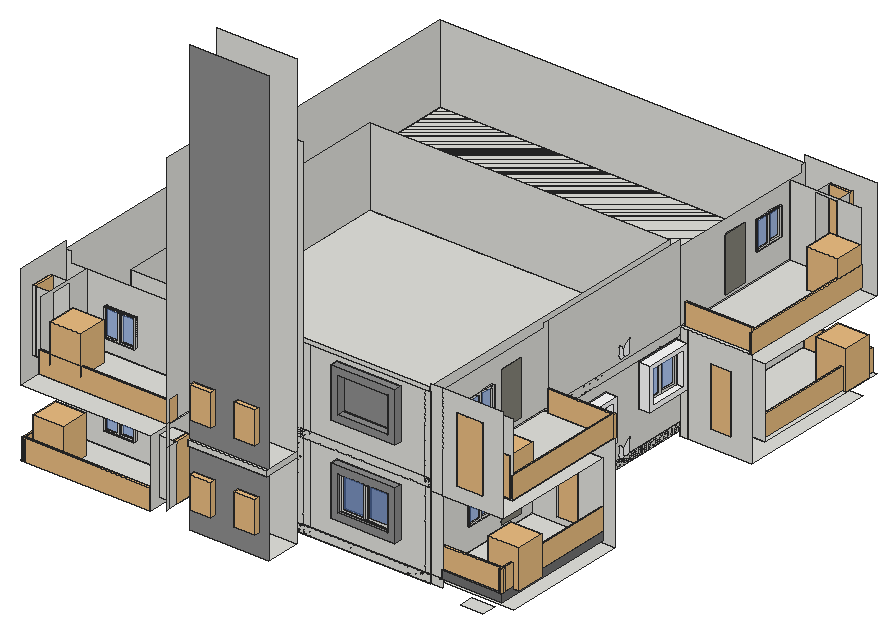
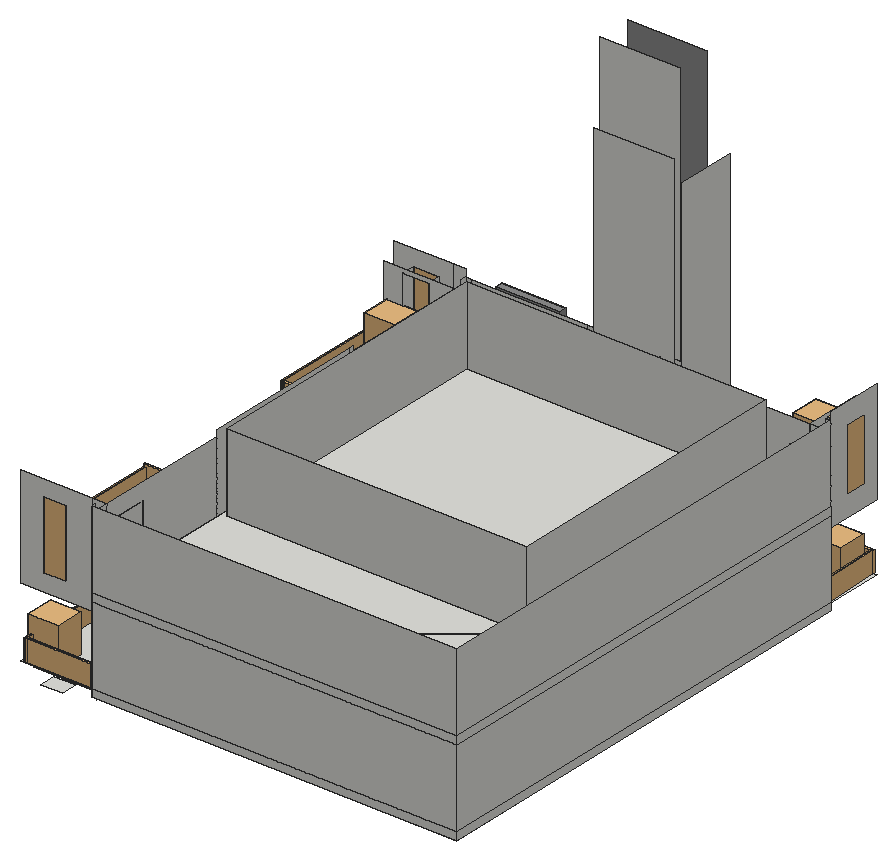
# SketchUp Ruby script. Lengths in inches.
U = 1.inch
M = Sketchup.active_model
def pt(a) = Geom::Point3d.new(a.map { |v| v * U })
def face(e, loops, mat)
  f = e.add_face(loops[0].map { |a| pt(a) })
  loops[1..].each { |l| e.add_face(l.map { |a| pt(a) }).erase! }
  f.material = f.back_material = mat if mat
  f
end
# faces: each face lists its corners as indices into pts; further lists are holes
def faces(e, pts, list, mat = nil) = list.each { |f| face(e, (f[0].is_a?(Array) ? f : [f]).map { |l| l.map { |i| pts[i] } }, mat) }
# xy, xz, yz: faces in a plane at the given z, y or x. An outline is a flat list of corners, or four numbers for a rectangle; further outlines are holes
def ring(l) = l.size == 4 ? [[l[0], l[1]], [l[2], l[1]], [l[2], l[3]], [l[0], l[3]]] : l.each_slice(2).to_a
def flat(e, list, mat, &to3) = list.each { |f| face(e, (f[0].is_a?(Array) ? f : [f]).map { |l| ring(l).map { |u, v| to3.(u, v) } }, mat) }
def xy(e, z, list, mat = nil) = flat(e, list, mat) { |x, y| [x, y, z] }
def xz(e, y, list, mat = nil) = flat(e, list, mat) { |x, z| [x, y, z] }
def yz(e, x, list, mat = nil) = flat(e, list, mat) { |y, z| [x, y, z] }
def lines(e, pts, list) = list.each { |a, b| e.add_line(pt(pts[a]), pt(pts[b])) }
# prism: a flat outline (further loops are holes) pulled along v
def prism(e, loops, v, mat = nil)
  f = face(e, loops, mat); d = Geom::Vector3d.new(v.map { |x| x * U })
  f.pushpull(f.normal.samedirection?(d) ? d.length : -d.length)
end
def box(e, o, s, mat = nil) = prism(e, [[o, [o[0] + s[0], o[1], o[2]], [o[0] + s[0], o[1] + s[1], o[2]], [o[0], o[1] + s[1], o[2]]]], [0, 0, s[2]], mat)
def at(x, y, z, deg = 0) = Geom::Transformation.translation(pt([x, y, z])) * Geom::Transformation.rotation(ORIGIN, Z_AXIS, deg.degrees)
def axes(o, x, y, z) = Geom::Transformation.new([*x, 0, *y, 0, *z, 0, *pt(o).to_a, 1])
def part(name) = M.definitions.add(name)
# library, detail: a bought-in or finely detailed component or shape, given as its bounding box
def library(name, o, s) = part(name).tap { |d| box(d.entities, o, s) }
def detail(e, o, s) = box(e.add_group.entities, o, s)
def put(e, d, t, mat = nil) = e.add_instance(d, t).tap { |i| i.material = mat if mat }
def group(e, t, mat = nil) = e.add_group.tap { |g| g.transformation = t; g.material = mat if mat }.entities
root = M.entities
M.materials.add("[Color C05]").color = [255, 127, 0]
M.materials.add("[Color M00]").color = [255, 255, 255]
M.materials.add("[Color M04]").color = [142, 142, 142]
M.materials.add("[Color M05]").color = [114, 114, 114]
M.materials.add("[Translucent Glass Blue]").color = [100, 149, 237]
M.materials["[Translucent Glass Blue]"].alpha = 0.5
M.materials.add("pic").color = [134, 132, 121]
c1 = library("KentiaPalm",[-22.86,-14.31,0],[47.49,43.96,59.125])
c2 = library("grade+varanda",[25.2,-1.57,0],[92.91,3.14,40.94])
c3 = part("Door leaf")
xy(c3.entities,0,[[0,0,28.74,2]],"pic")
xy(c3.entities,75.2,[[0,0,28.74,2]],"pic")
xz(c3.entities,0,[[0,0,28.74,75.2]],"pic")
xz(c3.entities,2,[[0,0,28.74,75.2]],"pic")
yz(c3.entities,0,[[0,0,2,75.2]])
yz(c3.entities,28.74,[[0,0,2,75.2]])
c4 = library("CNC CUTTING TEXTURE",[0,0,-0.79],[85.98,295.47,0.79])
c5 = library("Framed window",[0,0,0],[23.62,8.27,35.43])
c6 = part("Janela aluminio")
xy(c6.entities,0,[[0,0,47.24,1.57],[23.62,1.57,47.24,2.76],[0,2.76,25.98,3.9375],[0,3.9375,47.24,5.91]])
xy(c6.entities,43.31,[[0,0,47.24,1.57],[23.62,1.57,47.24,2.76],[0,2.76,0,5.91,47.24,5.91,47.24,3.9375,25.98,3.9375,25.98,2.76],[25.98,2.76,47.24,3.9375]])
xz(c6.entities,1.57,[[0,0,23.62,0,23.62,41.34,21.26,41.34,21.26,1.97,1.97,1.97,1.97,41.34,23.62,41.34,23.62,43.31,0,43.31],[[23.62,0,47.24,43.31],[25.7,1.97,45.28,41.34]]])
xz(c6.entities,2.76,[[[0,0,23.62,43.31],[2.36,2.36,21.26,40.94]],[23.62,0,25.98,43.31]])
xz(c6.entities,2.76,[[2.36,2.36,21.26,40.94]],"[Translucent Glass Blue]")
xz(c6.entities,3.9375,[[25.98,0,25.98,2.36,44.88,2.36,44.88,40.94,25.98,40.94,25.98,43.31,47.24,43.31,47.24,0]])
xz(c6.entities,3.9375,[[25.98,2.36,44.88,40.94]],"[Translucent Glass Blue]")
yz(c6.entities,0,[[0,0,1.57,43.31],[2.76,0,5.91,43.31]])
yz(c6.entities,23.62,[[1.57,0,2.76,43.31]])
yz(c6.entities,25.98,[[2.76,0,3.9375,43.31]])
yz(c6.entities,47.24,[[0,0,1.57,43.31],[1.57,0,2.76,43.31],[3.9375,0,5.91,43.31]])
c7 = part("Group\#81")
xy(c7.entities,0,[[[0,0,99.375,76.3125],[10.74,10.74,88.63,65.57]],[10.74,10.74,88.63,65.57]])
xy(c7.entities,11.8125,[[[0,0,99.375,76.3125],[10.74,10.74,88.63,65.57]]])
xz(c7.entities,0,[[0,0,99.375,11.8125]])
xz(c7.entities,10.74,[[10.74,0,88.63,11.8125]])
xz(c7.entities,65.57,[[10.74,0,88.63,11.8125]])
xz(c7.entities,76.3125,[[0,0,99.375,11.8125]])
yz(c7.entities,0,[[0,0,76.3125,11.8125]])
yz(c7.entities,10.74,[[10.74,0,65.57,11.8125]])
yz(c7.entities,88.63,[[10.74,0,65.57,11.8125]])
yz(c7.entities,99.375,[[0,0,76.3125,11.8125]])
c8 = part("Group\#73")
xy(c8.entities,0,[[6.22,6.22,66.16,57.66]],"[Color M00]")
xy(c8.entities,0,[[[0,0,72.375,63.875],[6.22,6.22,66.16,57.66]]],"[Color M04]")
xy(c8.entities,16.6875,[[[0,0,72.375,63.875],[6.22,6.22,66.16,57.66]]],"[Color M00]")
xz(c8.entities,0,[[0,0,72.375,16.6875]],"[Color M00]")
xz(c8.entities,6.22,[[6.22,0,66.16,16.6875]],"[Color M00]")
xz(c8.entities,57.66,[[6.22,0,66.16,16.6875]],"[Color M04]")
xz(c8.entities,63.875,[[0,0,72.375,16.6875]],"[Color M00]")
yz(c8.entities,0,[[0,0,63.875,16.6875]],"[Color M00]")
yz(c8.entities,6.22,[[6.22,0,57.66,16.6875]],"[Color M00]")
yz(c8.entities,66.16,[[6.22,0,57.66,16.6875]],"[Color M00]")
yz(c8.entities,72.375,[[0,0,63.875,16.6875]],"[Color M00]")
xy(root,277.65,[[815.15,221.79,849.53,244.2]])
xy(root,281.18,[[448.85,157.26,571.01,210.63]])
xy(root,281.29,[[813.66,917.62,847.23,942.88]])
xy(root,283.71,[[769.63,702.05,769.63,917.62,879.32,917.62,879.32,702.13,780.63,702.13,780.63,702.05]])
xy(root,284.02,[[769.63,244.2,879.32,439.19]])
xy(root,291.08,[[[206.95,222.13,769.63,942.88],[298.63,231.13,760.63,693.13]]])
xy(root,303.08,[[206.95,133.63,408.57,222.13],[769.63,221.79,786.7,222.13],[786.7,221.79,879.32,221.79,879.32,415.6,867.32,415.6,867.32,232.67,786.7,232.67],[[206.95,222.13,769.63,942.88],[298.63,231.13,760.63,693.13]],[769.63,222.13,786.7,222.13,786.7,232.67,867.32,232.67,867.32,415.6,769.63,415.6],
  [298.63,231.13,760.63,693.13],[769.63,728.91,879.32,942.88]])
xy(root,310.63,[[816.63,702.13,847.63,728.91]])
xy(root,311.64,[[808.92,415.6,840.79,439.19]])
xy(root,315.48,[[408.57,149.23,436.38,173.48]])
xy(root,316.02,[[786.7,221.79,879.32,221.79,879.32,415.6,867.32,415.6,867.32,232.67,786.7,232.67]],"[Color M05]")
xy(root,399.95,[[816.63,702.13,847.63,728.91]])
xy(root,402.1,[[408.57,149.23,436.38,173.48]])
xy(root,406.33,[[206.95,133.63,408.57,222.13]])
xy(root,407.95,[[808.92,415.6,840.79,439.19]])
xy(root,410.02,[[769.63,728.91,879.32,942.88]])
xy(root,418.39,[[769.63,222.13,879.32,415.6]])
xy(root,423.08,[[[206.95,222.13,769.63,942.88],[298.63,231.13,760.63,693.13]]])
xy(root,435.08,[[237.95,133.63,436.38,222.13],[[206.95,222.13,769.63,942.88],[298.63,231.13,760.63,693.13]],[298.63,231.13,760.63,693.13],[769.63,242.1,879.32,439.19],[769.63,702.05,780.63,702.05,780.63,702.13,879.32,702.13,879.32,913.11,769.63,913.11]])
xy(root,437.55,[[809.28,913.11,842.4,942.88]])
xy(root,438.3,[[206.95,156.57,237.95,190.94]])
xy(root,440.0625,[[810.64,222.13,849.77,242.1]])
xz(root,149.23,[[408.57,315.48,436.38,402.1]])
xz(root,156.57,[[206.95,438.3,237.95,534.42]])
xz(root,157.26,[[448.85,281.18,571.01,951.08]],"[Color M04]")
xz(root,173.48,[[408.57,315.48,436.38,402.1]])
xz(root,190.94,[[206.95,438.3,237.95,534.42]])
xz(root,210.63,[[448.85,281.18,571.01,951.08]])
xz(root,221.79,[[786.7,303.08,879.32,316.02]],"[Color M05]")
xz(root,222.13,[[206.95,291.08,436.38,303.08],[436.38,291.08,448.85,303.08],[448.85,291.08,571.01,831.08],[571.01,291.08,582.45,303.08],[582.45,291.08,759.63,303.08],
  [759.63,291.08,787.51,303.08],[206.95,303.08,408.57,406.33],[408.57,303.08,436.38,303.08,436.38,423.08,425.76,423.08,425.76,406.33,408.57,406.33],[436.38,303.08,448.85,423.08],[448.85,303.08,571.01,423.08],
  [571.01,303.08,582.45,423.08],[582.45,303.08,759.63,423.08],[759.63,303.08,769.63,423.08],[769.63,303.08,787.51,418.39],[206.95,406.33,425.76,423.08],
  [769.63,418.39,787.51,567.08],[[787.51,418.39,879.32,567.08],[810.64,440.0625,849.77,541.5625]],[206.95,423.08,436.38,435.08],[436.38,423.08,448.85,435.08],[571.01,423.08,582.45,435.08],
  [582.45,423.08,759.63,435.08],[759.63,423.08,769.63,435.08],[206.95,435.08,237.95,435.08,237.95,538.83,213.89,538.83,213.89,555.08,206.95,555.08],[237.95,435.08,436.38,435.08,436.38,555.08,435.45,555.08,435.45,538.83,237.95,538.83],[436.38,435.08,448.85,555.08],
  [448.85,435.08,571.01,555.08],[571.01,435.08,582.45,555.08],[582.45,435.08,759.63,555.08],[759.63,435.08,769.63,555.08]])
xz(root,231.13,[[298.63,303.08,760.63,423.08],[298.63,435.08,760.63,555.08]])
xz(root,232.67,[[786.7,303.08,867.32,316.02]])
xz(root,242.1,[[[769.63,435.08,879.32,548.14],[810.64,440.0625,849.77,541.5625]]])
xz(root,415.6,[[[769.63,303.08,867.32,303.08,867.32,316.02,879.32,316.02,879.32,418.39,769.63,418.39],[808.92,311.64,840.79,407.95]],[867.32,303.08,879.32,316.02]])
xz(root,439.19,[[[769.63,284.02,879.32,435.08],[808.92,311.64,840.79,407.95]]])
xz(root,693.13,[[298.63,303.08,760.63,423.08],[298.63,435.08,760.63,555.08]])
xz(root,702.05,[[769.63,283.71,780.63,435.08]])
xz(root,702.13,[[[780.63,283.71,879.32,435.08],[816.63,310.63,847.63,399.95]]])
xz(root,728.91,[[[769.63,303.08,879.32,410.02],[816.63,310.63,847.63,399.95]]])
xz(root,913.11,[[[769.63,435.08,879.32,545.21],[809.28,437.55,842.4,541.92]]])
xz(root,942.88,[[206.95,303.08,769.63,423.08],[[769.63,410.02,879.32,567.08],[809.28,437.55,842.4,541.92]],[206.95,435.08,769.63,555.08]])
yz(root,206.95,[[222.13,303.08,942.88,423.08],[[133.63,406.33,222.13,567.08],[156.57,438.3,190.94,534.42]],[222.13,435.08,942.88,555.08]])
yz(root,237.95,[[[133.63,435.08,222.13,538.83],[156.57,438.3,190.94,534.42]]])
yz(root,298.63,[[231.13,303.08,693.13,423.08],[231.13,435.08,693.13,555.08]])
yz(root,408.57,[[[133.63,303.08,222.13,406.33],[149.23,315.48,173.48,402.1]]])
yz(root,436.38,[[129.69,315.48,133.63,402.1],[133.63,315.48,149.23,402.1],[149.23,315.48,173.48,402.1],[129.69,402.1,133.63,435.08],[129.69,435.08,222.13,802.33]])
yz(root,760.63,[[231.13,303.08,693.13,423.08],[231.13,435.08,693.13,555.08]])
yz(root,769.63,[[702.05,283.71,702.13,291.08],[702.13,283.71,933.12,291.08],[244.2,284.02,431.41,284.02,431.41,291.08,238.89,291.08,238.89,287.21,244.2,287.21],[431.41,284.02,439.19,291.08],[447.18,291.08,702.05,303.08],
  [702.05,291.08,702.13,303.08],[702.13,291.08,942.88,303.08],[222.13,303.08,415.6,418.39],[415.6,303.08,439.19,423.08],[439.19,303.08,447.18,423.08],
  [447.18,303.08,702.05,423.08],[702.05,303.08,702.13,423.08],[702.13,303.08,728.91,303.08,728.91,410.02,706.6,410.02,706.6,423.08,702.13,423.08],[728.91,303.08,942.88,410.02],[706.6,410.02,942.88,423.08],
  [222.13,418.39,230.73,423.08],[230.73,418.39,415.6,423.08],[222.13,423.08,439.19,435.08],[447.18,423.08,702.05,435.08],[702.05,423.08,702.13,435.08],
  [702.13,423.08,942.88,435.08],[222.13,435.08,242.1,435.08,242.1,548.14,230.73,548.14,230.73,555.08,222.13,555.08],[242.1,435.08,447.18,435.08,447.18,555.08,439.19,555.08,439.19,548.14,242.1,548.14],[447.18,435.08,702.13,555.08],[702.13,435.08,913.11,545.21],
  [913.11,435.08,942.88,435.08,942.88,555.08,936.3,555.08,936.3,545.21,913.11,545.21]])
yz(root,780.63,[[577.58,312.75,578.17,313.28,578.83,313.81,579.23,314.54,579.45,315.36,579.62,316.22,578.67,318.28,578.48,319.05,578.04,319.73,578.04,320.54,578.03,321.45,577.98,322.25,577.92,323.22,577.81,323.98,577.48,324.74,577.16,325.41,576.92,326.28,576.64,327.1,576.3,327.8,575.73,328.48,575.21,328.93,574.43,329.6,573.76,330.23,572.95,330.52,572.6875,331.08,571.06,331.66,571,329.79,571.5,328.1,571.63,326.41,571.52,325.79,571.55,324.99,571.54,324.15,571.52,323.39,571.5,322.62,571.36,321.51,571.1,320.8,571.01,319.79,570.9375,318.95,570.87,318.04,571.05,317.33,571.28,316.55,571.66,315.77,572.09,314.89,572.79,314.43,573.44,313.82,574.125,313.32,574.95,313.11,575.7,312.94,576.67,312.82],[587.71,313.43,588.31,313.98,588.74,314.66,589.32,315.3,589.55,316.125,589.71,317,589.84,318.01,589.91,318.84,589.97,319.76,590.01,320.82,590.04,321.66,590.07,322.6,590.09,323.55,590.11,324.25,590.13,325.04,590.03,325.82,590.03,326.58,589.7,327.57,589.63,328.49,589.59,329.3,589.56,330.22,589.55,331.14,589.56,332.0625,589.65,332.64,589.35,332.39,588.79,332.32,588.13,331.9375,587.47,331.41,586.76,331.04,586.15,330.53,585.43,330.125,584.71,329.62,583.98,329.21,583.01,328.48,582.55,327.79,581.94,327.32,581.45,326.63,581.12,325.93,580.71,325.22,580.42,324.375,580.27,323.5,580.16,322.6,579.97,321.68,579.89,320.75,579.83,320.04,579.78,319.25,579.62,316.22,581.3,314.68,582.77,313.7,584.45,313.47,584.98,313.59,585.85,313.49,586.81,313.44],[577.58,450.3125,578.17,450.84,578.83,451.38,579.23,452.1,579.45,452.92,579.62,453.79,578.67,455.84,578.48,456.61,578.04,457.29,578.04,458.11,578.03,459.01,577.98,459.8125,577.92,460.79,577.81,461.55,577.48,462.31,577.16,462.98,576.92,463.84,576.64,464.66,576.3,465.36,575.73,466.04,575.21,466.49,574.43,467.16,573.76,467.79,572.95,468.08,572.6875,468.64,571.06,469.22,571,467.36,571.5,465.67,571.63,463.98,571.52,463.35,571.55,462.55,571.54,461.71,571.52,460.95,571.5,460.18,571.36,459.07,571.1,458.36,571.01,457.35,570.9375,456.51,570.87,455.6,571.05,454.89,571.28,454.11,571.66,453.33,572.09,452.45,572.79,451.99,573.44,451.38,574.125,450.89,574.95,450.67,575.7,450.51,576.67,450.39],[587.71,450.99,588.31,451.54,588.74,452.22,589.32,452.86,589.55,453.6875,589.71,454.56,589.84,455.57,589.91,456.4,589.97,457.32,590.01,458.38,590.04,459.22,590.07,460.16,590.09,461.11,590.11,461.82,590.13,462.6,590.03,463.38,590.03,464.14,589.7,465.13,589.63,466.05,589.59,466.86,589.56,467.78,589.55,468.71,589.56,469.625,589.65,470.2,589.35,469.95,588.79,469.88,588.13,469.5,587.47,468.97,586.76,468.6,586.15,468.1,585.43,467.6875,584.71,467.18,583.98,466.77,583.01,466.04,582.55,465.35,581.94,464.88,581.45,464.2,581.12,463.49,580.71,462.78,580.42,461.9375,580.27,461.06,580.16,460.16,579.97,459.24,579.89,458.31,579.83,457.6,579.78,456.82,579.62,453.79,581.3,452.25,582.77,451.26,584.45,451.03,584.98,451.16,585.85,451.05,586.81,451.01]],"[Color M00]")
yz(root,780.63,[[702.05,283.71,702.13,435.08],[589.65,332.64,590.67,333.5,591.45,335,589.67,332.77],[589.65,470.2,590.67,471.07,591.45,472.56,589.67,470.33]],"[Color M04]")
yz(root,786.7,[[221.79,303.08,232.67,316.02]])
yz(root,808.92,[[415.6,311.64,439.19,407.95]])
yz(root,809.28,[[913.11,437.55,942.88,541.92]])
yz(root,810.64,[[222.13,440.0625,242.1,541.5625]])
yz(root,816.63,[[702.13,310.63,728.91,399.95]])
yz(root,840.79,[[415.6,311.64,439.19,407.95]])
yz(root,842.4,[[913.11,437.55,942.88,541.92]])
yz(root,847.63,[[702.13,310.63,728.91,399.95]])
yz(root,849.77,[[222.13,440.0625,242.1,541.5625]])
yz(root,867.32,[[232.67,303.08,415.6,316.02]])
yz(root,879.32,[[221.79,303.08,415.6,316.02]],"[Color M05]")
p = [[780.63,578.67,455.84],[780.63,579.08,455.1875],[780.63,569.41,469.24],[780.63,571.06,469.22],[780.63,578.67,318.28],[780.63,579.08,317.625],
  [780.63,569.41,331.68],[780.63,571.06,331.66]]
lines(root,p,[[0,1],[2,3],[4,5],[6,7]])
g1 = group(root,at(289.63,702.13,291.08))
box(g1,[-82.6875,-480,0],[562.6875,720.75,12])
put(root,c1,at(238.42,160.96,302.87))
put(root,c1,at(854.6875,899.22,303.08))
put(root,c2,axes([209.39,244.3,303.08],[0.02789,-0.93959,0],[0.99956,0.02967,0],[0,0,0.8]))
put(root,c2,axes([157.3,134.04,303.22],[2.12,0,0],[0,1,0],[0,0,0.8]))
put(root,c2,axes([743.65,939.6,303.29],[1.0998,0,0],[0,1,0],[0,0,0.8]))
put(root,c2,axes([872.12,672.85,303.67],[0,2.2896,0],[-1,0,0],[0,0,0.8]))
put(root,c3,axes([367.18,217.42,304.02],[1.26,0,0],[0,1,0],[0,0,1.1]))
put(root,c3,axes([771.63,787.51,307.24],[0,1.26,0],[-1,0,0],[0,0,1.1]))
put(root,c4,axes([816.63,717.68,310.63],[0.36053,0,0],[0,0,0.30227],[0,19.75175,0]))
put(root,c4,axes([808.92,420.4,311.4375],[0.37071,0,0],[0,0,0.32664],[0,4.90816,0]),"[Color C05]")
put(root,c3,axes([771.63,355.51,313.47],[0,1.26,0],[-1,0,0],[0,0,1.1]))
put(root,c1,at(863.43,257.21,313.77))
put(root,c4,axes([431.38,149.23,315.73],[0,0.28203,0],[0,0,0.29233],[-6.34963,0,0]))
put(root,c2,axes([761.5,225.65,316.02],[1,0,0],[0,1,0],[0,0,0.8]))
put(root,c2,axes([877.75,165.21,317.01],[0,2.12,0],[-1,0,0],[0,0,0.8]))
put(root,c5,axes([529.875,141.71,319.89],[1.35,0,0],[0,1,0],[0,0,1.38]))
put(root,c5,axes([461.6875,141.71,319.89],[1.35,0,0],[0,1,0],[0,0,1.38]))
put(root,c6,at(269.17,216.22,329.09))
put(root,c6,at(774.2,845.05,336.54,90))
put(root,c7,axes([630.14,214.57,340.54],[1,0,0],[0,0,1],[0,-1,0]),"[Color M04]")
put(root,c6,at(774.2,290.89,340.61,90))
put(root,c6,axes([720.02,213.44,351.94],[-1.675,0,0],[0,-1,0],[0,0,1.25072]))
put(root,c8,axes([780.82,472.87,353.36],[0,1,0],[0,0,1],[1,0,0]),"[Color M00]")
put(root,c6,axes([785.51,479.08,359.58],[0,1.25,0],[-1,0,0],[0,0,1.1998]))
put(root,c8,axes([780.63,608.66,366.91],[0,1,0],[0,0,1],[1,0,0]),"[Color M00]")
put(root,c6,axes([786.92,614.88,373.125],[0,1.25,0],[-1,0,0],[0,0,1.1998]))
g2 = group(root,at(448.85,210.63,399.28))
box(g2,[0,-57.1875,0],[122.16,57.1875,8.15])
g3 = group(root,at(289.63,702.13,423.08))
box(g3,[-82.6875,-480,0],[562.6875,720.75,12])
put(root,c3,axes([367.18,217.42,430.33],[1.26,0,0],[0,1,0],[0,0,1.1]))
put(root,c2,axes([877.83,646.02,433.82],[0,2.2684,0],[-1,0,0],[0,0,0.8]))
put(root,c2,axes([431.96,244.65,434.39],[0.02789,-0.93959,0],[0.99956,0.02967,0],[0,0,0.8]))
put(root,c2,axes([184.53,132.06,434.48],[2.12,0,0],[0,1,0],[0,0,0.8]))
put(root,c1,at(854.6875,883.32,435.08))
put(root,c2,axes([750.15,437.71,436.27],[1.0998,0,0],[0,1,0],[0,0,0.8]))
put(root,c2,axes([877.75,188.6875,436.62],[0,2.12,0],[-1,0,0],[0,0,0.8]))
put(root,c1,at(850.68,255.8,437.11))
put(root,c4,axes([809.28,942.88,437.55],[0.38524,0,0],[0,0,0.35325],[0,6.12304,0]))
put(root,c4,axes([206.95,156.57,438.3],[0,0.39978,0],[0,0,0.32533],[-6.34963,0,0]))
put(root,c2,axes([749.5,703.75,438.62],[1.0998,0,0],[0,1,0],[0,0,0.8]))
put(root,c4,axes([810.64,221.19,440.0625],[0.45503,0,0],[0,0,0.34352],[0,-1.1913,0]))
put(root,c3,axes([771.63,787.51,442.3],[0,1.26,0],[-1,0,0],[0,0,1.1]))
put(root,c5,axes([461.6875,141.71,443.71],[1.35,0,0],[0,1,0],[0,0,1.38]))
put(root,c5,axes([529.875,141.71,443.71],[1.35,0,0],[0,1,0],[0,0,1.38]))
put(root,c3,axes([771.63,355.51,446.1],[0,1.26,0],[-1,0,0],[0,0,1.1]))
put(root,c1,at(277.49,145.94,452.43))
put(root,c6,at(269.17,216.22,456.9))
put(root,c6,at(774.2,291.2,472.11,90))
put(root,c7,axes([630.14,214.57,476.29],[1,0,0],[0,0,1],[0,-1,0]),"[Color M04]")
put(root,c6,at(774.2,845.05,477.11,90))
